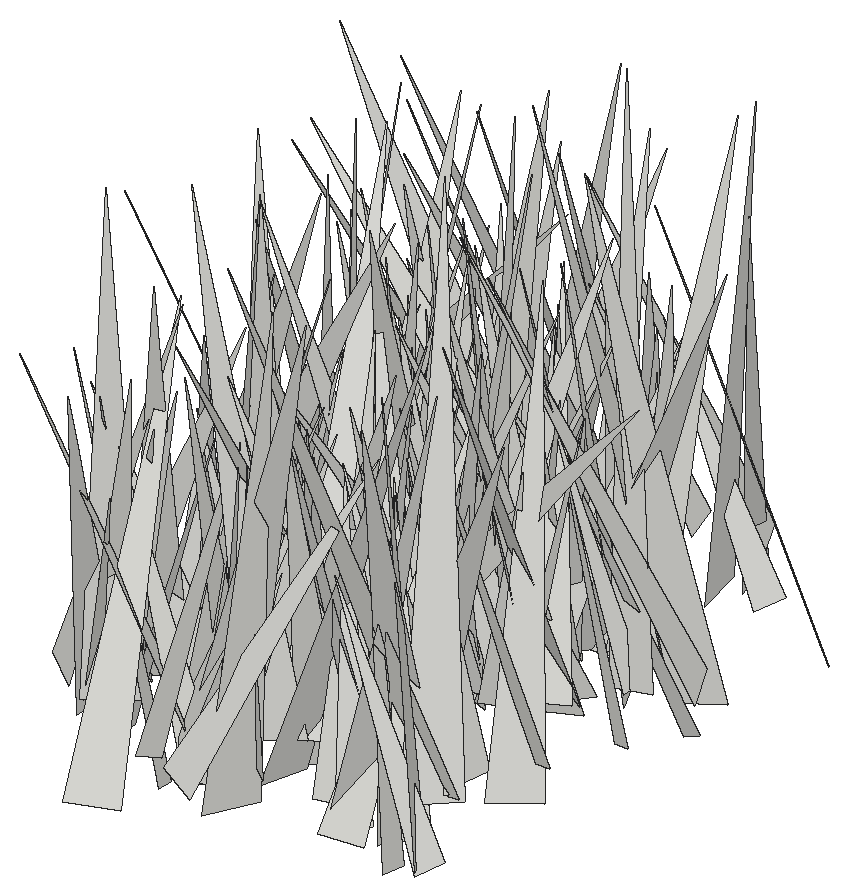
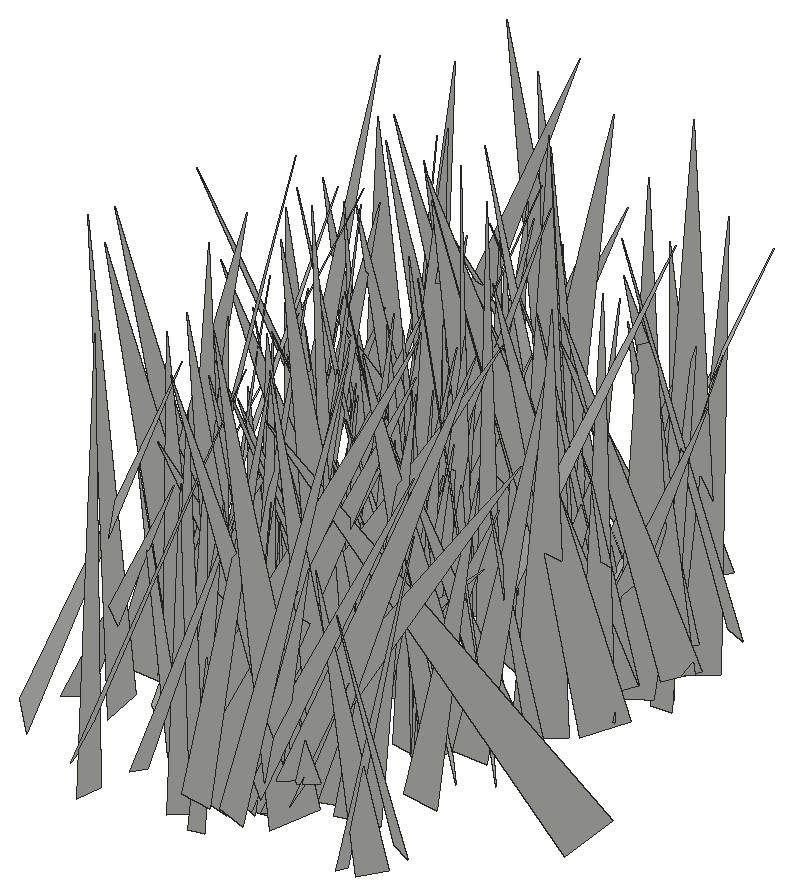
# SketchUp Ruby script. Lengths in inches.
U = 1.inch
M = Sketchup.active_model
def pt(a) = Geom::Point3d.new(a.map { |v| v * U })
def face(e, loops, mat)
  f = e.add_face(loops[0].map { |a| pt(a) })
  loops[1..].each { |l| e.add_face(l.map { |a| pt(a) }).erase! }
  f.material = f.back_material = mat if mat
  f
end
# faces: each face lists its corners as indices into pts; further lists are holes
def faces(e, pts, list, mat = nil) = list.each { |f| face(e, (f[0].is_a?(Array) ? f : [f]).map { |l| l.map { |i| pts[i] } }, mat) }
# xy, xz, yz: faces in a plane at the given z, y or x. An outline is a flat list of corners, or four numbers for a rectangle; further outlines are holes
def ring(l) = l.size == 4 ? [[l[0], l[1]], [l[2], l[1]], [l[2], l[3]], [l[0], l[3]]] : l.each_slice(2).to_a
def flat(e, list, mat, &to3) = list.each { |f| face(e, (f[0].is_a?(Array) ? f : [f]).map { |l| ring(l).map { |u, v| to3.(u, v) } }, mat) }
def xy(e, z, list, mat = nil) = flat(e, list, mat) { |x, y| [x, y, z] }
def xz(e, y, list, mat = nil) = flat(e, list, mat) { |x, z| [x, y, z] }
def yz(e, x, list, mat = nil) = flat(e, list, mat) { |y, z| [x, y, z] }
def lines(e, pts, list) = list.each { |a, b| e.add_line(pt(pts[a]), pt(pts[b])) }
# prism: a flat outline (further loops are holes) pulled along v
def prism(e, loops, v, mat = nil)
  f = face(e, loops, mat); d = Geom::Vector3d.new(v.map { |x| x * U })
  f.pushpull(f.normal.samedirection?(d) ? d.length : -d.length)
end
def box(e, o, s, mat = nil) = prism(e, [[o, [o[0] + s[0], o[1], o[2]], [o[0] + s[0], o[1] + s[1], o[2]], [o[0], o[1] + s[1], o[2]]]], [0, 0, s[2]], mat)
def at(x, y, z, deg = 0) = Geom::Transformation.translation(pt([x, y, z])) * Geom::Transformation.rotation(ORIGIN, Z_AXIS, deg.degrees)
def axes(o, x, y, z) = Geom::Transformation.new([*x, 0, *y, 0, *z, 0, *pt(o).to_a, 1])
def part(name) = M.definitions.add(name)
# library, detail: a bought-in or finely detailed component or shape, given as its bounding box
def library(name, o, s) = part(name).tap { |d| box(d.entities, o, s) }
def detail(e, o, s) = box(e.add_group.entities, o, s)
def put(e, d, t, mat = nil) = e.add_instance(d, t).tap { |i| i.material = mat if mat }
def group(e, t, mat = nil) = e.add_group.tap { |g| g.transformation = t; g.material = mat if mat }.entities
root = M.entities
c1 = part("fur_instance\#9")
p = [[0.8125,0,1.79],[0.67,-0.02,1.48],[0,-0.11,0],[0,0.11,0]]
faces(c1.entities,p,[[0,1,2,3]])
put(root,c1,axes([89.85,77.52,-28.22],[0.35019,4.61175,0.40741],[4.56098,-0.41379,0.76359],[-0.79477,-0.34263,4.56155]))
put(root,c1,axes([88.22,83.61,-27.1],[3.62066,0.28745,0.41277],[0.34104,-3.60783,-0.479],[-0.36973,-0.51296,3.60033]))
put(root,c1,axes([88.46,77.83,-28.22],[-1.94792,-5.41513,0.85515],[-5.11405,2.12183,1.78705],[1.97517,0.15336,5.47032]))
put(root,c1,axes([89.04,88.7,-28.22],[1.79566,3.71313,0.76849],[3.77743,-1.82574,-0.00496],[-0.33004,-0.69403,4.12452]))
put(root,c1,axes([90.1,81.2,-28.22],[-4.52139,5.22079,2.42729],[5.56937,4.74843,0.161],[1.45961,-1.94607,6.90462]))
put(root,c1,axes([91.15,77.77,-28.22],[-4.32688,2.05759,1.06704],[2.30248,4.07514,1.47851],[0.2661,-1.80382,4.55737]))
put(root,c1,axes([89.63,84.88,-27.1],[-0.57876,-6.04691,0.53315],[-6.05695,0.61084,0.35302],[0.40347,0.49606,6.06428]))
put(root,c1,axes([90.38,86.13,-28.22],[-0.10037,-5.00985,1.67679],[-5.24561,-0.10471,-0.62683],[-0.62754,1.67652,4.9715]))
put(root,c1,axes([87.71,81.27,-27.1],[5.60342,-3.67276,1.04707],[-3.81273,-5.48708,1.15708],[-0.22057,1.54484,6.59914]))
put(root,c1,axes([88.14,81.08,-27.1],[0.06322,-6.05576,0.15688],[-5.74231,-0.00994,1.93043],[1.92942,0.16885,5.74018]))
put(root,c1,axes([88.02,77.62,-27.1],[0.93957,-4.99379,0.05949],[-4.70596,-0.86502,1.71172],[1.67197,0.37157,4.78443]))
put(root,c1,axes([87.93,77.6,-27.1],[2.95683,-4.48742,1.40063],[-4.613,-2.45121,1.88504],[0.90496,2.16707,5.03253]))
put(root,c1,axes([88.21,74.84,-27.1],[3.54049,4.95211,1.34575],[5.12044,-3.30078,-1.32493],[0.33991,-1.85767,5.94164]))
put(root,c1,axes([89.72,90.47,-28.22],[-4.12038,-2.11418,1.50488],[-1.47976,4.23386,1.89649],[2.13184,-1.14743,4.225]))
put(root,c1,axes([88.83,75.66,-28.22],[6.03542,-2.39463,0.80521],[-2.12324,-5.9379,-1.74415],[-1.3691,-1.34759,6.25448]))
put(root,c1,axes([85.43,84.82,-28.22],[6.0984,-4.54505,0.22334],[-3.82324,-4.91501,4.37303],[2.46783,3.61705,6.22291]))
put(root,c1,axes([88.97,76.35,-27.1],[3.21186,-3.52218,0.8528],[-3.62385,-3.13,0.72104],[-0.02677,1.11644,4.71189]))
put(root,c1,axes([90.29,74.41,-27.1],[4.03772,-5.94106,3.0996],[-6.44975,-4.42725,-0.08397],[-1.8178,2.512,7.18278]))
put(root,c1,axes([89.54,74.5,-27.1],[3.73813,0.01426,0.67221],[0.17612,-3.68545,-0.90117],[-0.64889,-0.91811,3.62791]))
put(root,c1,axes([92.89,88.93,-28.22],[-7.69272,2.37823,1.5322],[2.71051,7.46743,2.01798],[0.8104,-2.40066,7.79498]))
put(root,c1,axes([89.15,77.73,-28.22],[4.02071,-6.30995,0.86141],[-6.36147,-4.02715,0.19326],[-0.29869,0.83076,7.47959]))
put(root,c1,axes([92.9,73.3,-28.22],[-5.46466,-2.11839,0.66349],[-2.21236,5.05235,-2.09036],[-0.18243,2.18553,5.47545]))
put(root,c1,axes([88.9,90.13,-28.22],[2.31724,-3.70248,0.25487],[-3.62607,-2.19471,1.08527],[0.79054,0.78602,4.23086]))
put(root,c1,axes([94.19,88.4,-28.22],[-2.35699,-6.63901,0.53799],[-6.01099,1.87426,-3.2057],[-2.86948,1.52709,6.27339]))
put(root,c1,axes([89.55,75.04,-27.1],[3.84963,-3.94903,0.87916],[-4.01863,-3.87266,0.20133],[-0.4673,0.77142,5.51126]))
put(root,c1,axes([89.84,83.51,-28.22],[5.88152,4.86813,2.28116],[5.13014,-6.09312,-0.22398],[-1.60749,-1.63397,7.63157]))
put(root,c1,axes([90.27,75.01,-28.22],[4.03699,1.00135,1.00845],[0.75439,-4.0837,1.03503],[-1.2044,0.79854,4.02849]))
put(root,c1,axes([93.26,80.22,-27.1],[-4.92734,-5.46841,0.2776],[-5.45988,4.87887,-0.80338],[-0.41255,0.74316,7.31688]))
put(root,c1,axes([93.45,89.71,-27.1],[-3.66042,-4.84933,0.70173],[-4.78346,3.34689,-1.82316],[-1.06154,1.63996,5.79575]))
put(root,c1,axes([89.6,83.15,-27.1],[4.44559,-0.41699,0.42413],[-0.48383,-4.39553,0.74982],[-0.34594,0.78895,4.4017]))
put(root,c1,axes([93.32,74.62,-28.22],[-5.39414,-3.77764,0.22745],[-3.78403,5.38986,-0.22257],[0.05845,0.31282,6.58162]))
put(root,c1,axes([91.07,88.09,-28.22],[1.80262,-6.00522,1.15434],[-6.08405,-1.88243,-0.2921],[-0.61598,1.01901,6.26312]))
put(root,c1,axes([91.19,76.49,-28.22],[3.26782,5.25044,1.3347],[5.28581,-3.43164,0.55786],[-1.18691,-0.82697,6.1591]))
put(root,c1,axes([92.125,71.23,-28.22],[-4.33285,5.33033,0.39838],[5.19442,4.31986,-1.30443],[1.26061,0.52067,6.74422]))
put(root,c1,axes([91.43,83.35,-28.22],[-4.86903,5.31705,1.90275],[5.12727,5.21523,-1.45307],[2.36698,-0.35954,7.06166]))
put(root,c1,axes([93.01,77.57,-28.22],[-1.35537,3.98703,1.26023],[4.07237,0.95801,1.34893],[-0.94888,-1.58348,3.98921]))
put(root,c1,axes([91.51,77.72,-27.1],[4.6906,-0.13116,1.94102],[0.35682,-4.92253,-1.19491],[-1.91244,-1.24013,4.53774]))
put(root,c1,axes([92.78,88.86,-28.22],[-3.67924,-0.76157,0.35539],[-0.68587,3.64327,0.70657],[0.48566,-0.62424,3.6902]))
put(root,c1,axes([93.61,81.77,-27.1],[-2.38468,3.13652,0.12042],[3.02513,2.25628,1.13874],[-0.83714,-0.7813,3.77197]))
put(root,c1,axes([93.64,73.99,-28.22],[-2.38269,3.95567,1.05235],[4.03891,2.07425,1.34786],[-0.66484,-1.57548,4.41677]))
put(root,c1,axes([90.74,84.18,-28.22],[-4.56158,-4.36485,4.54967],[-5.17144,5.80258,0.38189],[3.60662,2.79958,6.30192]))
put(root,c1,axes([88.87,79.65,-27.1],[4.47531,-6.51665,1.20055],[-6.35255,-3.80729,3.0143],[1.88498,2.64087,7.30815]))
put(root,c1,axes([92.51,84.03,-28.22],[-3.25997,-4.21096,1.97124],[-4.4396,3.53441,0.20814],[1.38129,1.42168,5.3213]))
put(root,c1,axes([92.71,91.65,-27.1],[-2.90954,-6.16313,0.64564],[-6.10361,2.97343,0.8781],[1.07095,0.20243,6.75859]))
put(root,c1,axes([93.57,84.49,-28.22],[-6.39617,-0.72322,1.67284],[-0.5993,6.59982,0.56183],[1.72113,-0.38959,6.41236]))
put(root,c1,axes([93.48,89.43,-28.22],[1.42744,-3.53628,2.17287],[-3.81125,-2.02664,-0.79456],[-1.64348,1.62839,3.72982]))
put(root,c1,axes([92.29,80.73,-28.22],[7.19679,1.10507,2.93039],[1.40985,-7.70082,-0.55845],[-2.79655,-1.03845,7.25969]))
put(root,c1,axes([92.34,85.6,-28.22],[4.23333,1.58778,2.03705],[2.11026,-4.38143,-0.97034],[-1.48911,-1.69519,4.41595]))
put(root,c1,axes([92.1,78.51,-27.1],[3.60415,-6.43604,2.10161],[-6.7075,-3.71823,0.11619],[-0.92131,1.89247,7.37557]))
put(root,c1,axes([89.6875,79.16,-28.22],[8.03575,1.73258,0.69022],[1.85682,-7.7181,-2.24381],[-0.17451,-2.34107,7.90825]))
put(root,c1,axes([96.3,86.22,-27.1],[-7.10232,2.48969,0.17848],[2.39972,6.66255,2.55443],[-0.68683,-2.46683,7.07929]))
put(root,c1,axes([92.89,72.65,-27.1],[-4.41851,1.16155,1.66424],[0.34777,4.36157,-2.12081],[1.99949,1.8082,4.04655]))
put(root,c1,axes([92.1,83.53,-28.22],[5.9168,-1.45412,1.7202],[-1.44139,-6.15974,-0.24915],[-1.73089,0.15879,6.08776]))
put(root,c1,axes([92.58,84.09,-28.22],[-1.22041,-5.00142,1.71972],[-5.19067,1.47111,0.5948],[1.01418,1.51086,5.11369]))
put(root,c1,axes([95.125,89.82,-28.22],[0.03934,-7.1777,0.79174],[-6.87762,-0.27857,-2.18369],[-2.20103,0.74216,6.83757]))
put(root,c1,axes([92.08,87.73,-28.22],[0.14436,6.2225,2.72909],[6.68972,0.34776,-1.14678],[1.18962,-2.71069,6.11762]))
put(root,c1,axes([93.19,78.625,-28.22],[-1.7362,-3.80786,1.79903],[-4.13168,1.91701,0.07019],[0.81577,1.60498,4.18441]))
put(root,c1,axes([96.39,82.44,-28.22],[-3.03964,-3.22245,0.08473],[-2.53096,2.3136,-2.80576],[-1.9964,1.97328,3.42802]))
put(root,c1,axes([92.57,80.72,-27.1],[3.35621,4.76804,0.53975],[4.75729,-3.3924,0.38655],[-0.62744,-0.21695,5.81798]))
put(root,c1,axes([93.99,85.64,-28.22],[-1.52023,5.3398,1.43684],[5.52962,1.4775,0.35965],[0.03531,-1.48075,5.54032]))
put(root,c1,axes([93.42,80.28,-27.1],[4.5767,5.68819,3.18986],[6.17982,-5.02762,0.09872],[-2.08339,-2.41752,7.30013]))
put(root,c1,axes([92.99,77.04,-27.1],[2.64907,4.14771,0.84835],[4.17625,-2.72433,0.27885],[-0.69438,-0.56151,4.91358]))
put(root,c1,axes([96.71,88.74,-28.22],[-3.02685,-7.70536,1.30124],[-7.48247,2.45538,-2.86554],[-2.25353,2.19686,7.76679]))
put(root,c1,axes([93.05,81.78,-27.1],[3.48904,-1.79502,0.75996],[-1.60226,-3.52839,-0.97792],[-1.11014,-0.54905,3.7999]))
put(root,c1,axes([94.92,75.38,-27.1],[1.79805,-6.87497,3.712],[-7.43664,-2.674,-1.35027],[-2.39594,3.14033,6.97674]))
put(root,c1,axes([94.07,74.16,-28.22],[-7.10447,-2.39928,3.44832],[-3.25719,7.42464,-1.54476],[2.65295,2.69055,7.33783]))
put(root,c1,axes([95.2,80.11,-27.1],[-4.58169,-0.00231,0.33908],[-0.10273,4.38765,-1.35823],[0.32316,1.36211,4.37574]))
put(root,c1,axes([93.87,89.46,-28.22],[-1.43466,-3.23484,0.82707],[-3.31328,1.49057,0.08262],[0.41278,0.72144,3.53774]))
put(root,c1,axes([93.36,81.81,-27.1],[0.28978,-3.77503,0.68612],[-3.83038,-0.24462,0.27184],[0.22308,0.70349,3.77636]))
put(root,c1,axes([92.47,89.13,-28.22],[7.15421,-1.9799,2.12173],[-2.22149,-7.36827,0.61487],[-1.86728,1.18029,7.39761]))
put(root,c1,axes([95.91,78,-28.22],[-0.66678,7.09806,0.59701],[6.83624,0.46921,2.05647],[-2.00116,-0.76214,6.82627]))
put(root,c1,axes([94.06,91.54,-27.1],[-1.823,-5.96341,0.88128],[-5.94354,1.93183,0.77754],[1.00658,0.60664,6.18716]))
put(root,c1,axes([96.38,80.29,-28.22],[-7.8071,-1.03462,1.04066],[-0.93299,7.84786,0.80297],[1.13267,-0.66693,7.83431]))
put(root,c1,axes([93.01,86.04,-27.1],[-2.73382,6.12597,3.74599],[6.6709,3.64992,-1.10045],[2.6569,-2.86083,6.61742]))
put(root,c1,axes([92.61,85.71,-27.1],[1.69765,-3.69471,0.41656],[-3.54176,-1.46758,1.41724],[1.13153,0.9496,3.81108]))
put(root,c1,axes([96.04,78.1,-27.1],[-1.10699,-6.38687,0.31821],[-6.26084,1.01671,-1.37367],[-1.30201,0.54128,6.33487]))
put(root,c1,axes([92.375,88.9375,-27.1],[1.25839,-5.65908,2.69216],[-6.0262,-0.33916,2.10388],[1.71982,2.95233,5.40207]))
put(root,c1,axes([95.6,75.94,-27.1],[-4.43994,6.98412,0.3729],[6.94517,4.45476,-0.74146],[0.82561,0.08476,8.24265]))
put(root,c1,axes([96.21,78.95,-27.1],[-2.14589,-4.13922,0.79032],[-4.13009,1.88974,-1.31675],[-0.83673,1.28775,4.4726]))
put(root,c1,axes([94.56,80.97,-27.1],[3.67967,2.76321,1.03507],[2.46473,-3.78797,1.35021],[-1.62229,0.51247,4.39911]))
put(root,c1,axes([93.76,82.29,-27.1],[0.23103,-4.99246,1.62863],[-5.17408,0.0623,0.92493],[0.89778,1.64376,4.91147]))
put(root,c1,axes([93.25,83.4375,-27.1],[6.31463,-5.10403,0.36931],[-4.97216,-6.25818,-1.47472],[-1.21044,-0.91981,7.98441]))
put(root,c1,axes([92.95,73.8,-27.1],[3.70587,4.25797,0.60198],[4.28884,-3.60158,-0.92773],[0.31394,-1.06043,5.56805]))
put(root,c1,axes([94.41,73.7,-27.1],[1.13394,4.06883,0.24777],[4.07369,-1.14042,0.08414],[-0.14769,-0.216,4.22305]))
put(root,c1,axes([93.99,87.58,-28.22],[3.64013,-0.49009,0.65042],[-0.33955,-3.62113,-0.82821],[-0.74023,-0.74902,3.57838]))
put(root,c1,axes([93.8125,74.01,-28.22],[4.14579,-2.60609,2.17076],[-3.31381,-3.84297,1.71517],[-0.72292,2.67047,4.58667]))
put(root,c1,axes([96.46,77.41,-28.22],[-5.48359,2.23586,1.70204],[2.68404,5.27249,1.72124],[0.83185,-2.27324,5.66623]))
put(root,c1,axes([93.81,78.3,-27.1],[5.31663,-1.02418,0.76649],[-0.77202,-5.18142,-1.56841],[-1.02002,-1.41668,5.18224]))
put(root,c1,axes([94.58,74.5,-27.1],[3.50873,2.55931,1.93983],[3.03472,-3.58228,-0.76287],[-1.05048,-1.80039,4.27543]))
put(root,c1,axes([95.61,81.625,-28.22],[3.52477,-3.78027,2.43443],[-3.94318,-4.08529,-0.63451],[-2.1606,1.28874,5.1295]))
put(root,c1,axes([97.88,79.3,-28.22],[-1.67581,5.69721,1.32161],[5.39716,0.9769,2.63242],[-2.25291,-1.89755,5.32325]))
put(root,c1,axes([96.53,86.07,-27.1],[-0.29394,-4.28793,0.2812],[-4.0742,0.18848,-1.38464],[-1.36614,0.36048,4.06885]))
put(root,c1,axes([96.42,81.74,-28.22],[-3.5063,-5.04513,2.56803],[-5.65565,3.25438,-1.32851],[0.24851,2.88062,5.99854]))
put(root,c1,axes([95.85,83.48,-27.1],[-3.35833,-3.2337,1.73378],[-3.57177,3.41915,-0.54142],[0.83981,1.61055,4.63056]))
put(root,c1,axes([94.2,91.33,-28.22],[3.64505,-0.39812,0.27738],[-0.20845,-3.18305,-1.82936],[-0.43816,-1.79764,3.17779]))
put(root,c1,axes([95.62,73.77,-27.1],[-2.49049,-3.07283,1.62396],[-3.33154,2.67981,-0.03854],[0.99012,1.28779,3.95516]))
put(root,c1,axes([96.83,80.66,-28.22],[-3.33504,1.53851,0.16438],[1.54705,3.32218,0.29368],[0.02564,-0.33558,3.66104]))
put(root,c1,axes([96.35,87.49,-27.1],[-3.41179,-1.77285,0.16017],[-1.67154,3.30984,1.02951],[0.61205,-0.84317,3.70451]))
put(root,c1,axes([95.3,87.68,-28.22],[-2.68709,-2.60275,1.28992],[-2.48203,2.97011,0.82256],[1.50922,0.25052,3.6494]))
put(root,c1,axes([94.3,78.03,-27.1],[-0.53016,-5.209,0.61736],[-4.97847,0.69512,1.58982],[1.65216,0.4231,4.98871]))
put(root,c1,axes([95.52,84.36,-27.1],[2.55514,-3.36467,0.69917],[-3.31318,-2.64324,-0.61213],[-0.91251,0.1757,4.18031]))
put(root,c1,axes([96.38,91.1875,-27.1],[-4.22859,-0.79072,0.99748],[-0.41595,4.12901,1.5098],[1.20299,-1.35177,4.02824]))
put(root,c1,axes([95.66,89.77,-27.1],[0.8315,-3.67241,0.7269],[-3.73531,-0.86356,-0.09004],[-0.24991,0.6885,3.76429]))
put(root,c1,axes([95.02,73.39,-28.22],[6.93717,-2.75986,2.51351],[-2.97128,-7.29338,0.19237],[-2.25967,1.11744,7.46352]))
put(root,c1,axes([95.38,76.72,-28.22],[3.36896,-5.0045,1.18358],[-5.04079,-3.49374,-0.42432],[-1.01802,0.73793,6.01788]))
put(root,c1,axes([96.93,83.9375,-27.1],[-5.40914,1.11965,1.3835],[1.23539,5.5484,0.3398],[1.28121,-0.62292,5.51334]))
put(root,c1,axes([93.54,74.89,-27.1],[5.39011,-5.98506,0.75501],[-6.02641,-5.29691,1.03406],[0.27067,1.25142,7.9878]))
put(root,c1,axes([94.32,80.53,-28.22],[3.5807,5.01538,0.32607],[5.01642,-3.54168,-0.61141],[0.30977,-0.61982,6.13202]))
put(root,c1,axes([93.57,77.95,-28.22],[3.71453,-6.09838,0.78607],[-6.05056,-3.46164,1.73599],[1.09493,1.55972,6.92635]))
put(root,c1,axes([95.15,83.68,-28.22],[4.01305,-1.4697,0.35123],[-1.33059,-3.90931,-1.15533],[-0.71618,-0.97223,4.11458]))
put(root,c1,axes([96.84,81.49,-27.1],[-5.64756,-4.03637,0.24701],[-3.60758,5.22048,2.82493],[1.82721,-2.16853,6.3409]))
put(root,c1,axes([95.04,90.76,-28.22],[3.21105,-3.45107,0.18225],[-3.45172,-3.21492,-0.06213],[-0.16965,0.09106,4.71348]))
put(root,c1,axes([96.62,82.15,-27.1],[3.17531,6.56755,2.54139],[6.79761,-3.58673,0.77578],[-1.83954,-1.91744,7.25351]))
put(root,c1,axes([95.5,89.71,-27.1],[-0.07367,-4.26522,0.50041],[-4.16979,0.19077,1.01214],[1.02732,0.46845,4.14405]))
put(root,c1,axes([95.33,90.36,-27.1],[0.2797,-5.08952,0.70223],[-5.01624,-0.11848,1.13926],[1.11073,0.74654,4.96825]))
put(root,c1,axes([94.34,71.99,-27.1],[1.81357,5.35205,0.20733],[5.12174,-1.66889,-1.72019],[1.56691,-0.73948,5.38279]))
put(root,c1,axes([97.3125,80.56,-27.1],[-0.77658,-4.10323,1.17838],[-4.23531,0.59015,-0.73621],[-0.53592,1.28194,4.11067]))
put(root,c1,axes([97.63,76.18,-28.22],[-2.42816,-5.42807,1.43938],[-5.61543,2.33238,-0.67728],[-0.05217,1.5899,5.90772]))
put(root,c1,axes([97.05,75.31,-28.22],[-1.64071,6.20292,1.41522],[6.35653,1.66047,0.09149],[0.27128,-1.39198,6.41559]))
put(root,c1,axes([95.48,85.72,-27.1],[5.08569,0.11573,0.95874],[0.07501,-5.17107,0.22632],[-0.96278,0.20845,5.08197]))
put(root,c1,axes([98.34,83.42,-28.22],[1.14957,-5.99203,1.40359],[-5.68779,-1.57972,-2.08556],[-2.35023,0.89221,5.73379]))
put(root,c1,axes([98.45,76.41,-28.22],[-5.17368,4.83178,0.63052],[4.85594,5.1888,0.08232],[0.40437,-0.49072,7.07858]))
put(root,c1,axes([98.26,91.62,-27.1],[-5.70608,-2.81682,0.48614],[-2.67601,5.6456,1.30244],[1.0049,-0.96065,6.22877]))
put(root,c1,axes([96.73,86.46,-27.1],[-3.34858,-4.98605,1.16696],[-4.83329,3.53804,1.24784],[1.69169,0.23891,5.87509]))
put(root,c1,axes([97.04,78.9,-27.1],[-3.71631,2.59474,2.95715],[3.6126,3.86147,1.15179],[1.55775,-2.76492,4.38373]))
put(root,c1,axes([95.0625,82.93,-28.22],[2.79379,4.96818,0.70977],[4.95175,-2.59669,-1.31495],[0.8165,-1.25148,5.54607]))
put(root,c1,axes([96.2,77.72,-28.22],[5.43956,-0.0104,1.6458],[0.01524,-5.68242,-0.08629],[-1.64576,-0.087,5.43889]))
put(root,c1,axes([97.13,85.77,-28.22],[-1.01475,7.09695,1.79918],[7.31311,1.06925,-0.09303],[0.3496,-1.76734,7.16853]))
put(root,c1,axes([95.45,83.1875,-27.1],[4.11337,-1.35782,0.42666],[-1.42017,-4.00175,0.95638],[-0.09392,1.04301,4.22479]))
put(root,c1,axes([96.54,85.43,-28.22],[-1.17903,-5.46423,1.73554],[-5.62366,1.44698,0.7353],[1.11548,1.51937,5.54141]))
put(root,c1,axes([98.17,74.54,-28.22],[-4.11869,2.39634,0.55767],[2.352,4.15398,-0.47915],[0.72219,0.13795,4.74094]))
put(root,c1,axes([95.05,75.52,-28.22],[7.44021,-1.05618,0.97458],[-1.13327,-7.472,0.55406],[-0.88376,0.68976,7.49435]))
put(root,c1,axes([95.67,81.49,-28.22],[-0.17372,7.00266,1.70424],[6.95108,0.61311,-1.81067],[1.90374,-1.5996,6.76675]))
put(root,c1,axes([96.63,78.625,-28.22],[4.55576,-0.64185,1.19418],[-0.37344,-4.61891,-1.05794],[-1.3033,-0.92017,4.47746]))
put(root,c1,axes([97.33,79.07,-27.1],[4.31579,6.0344,1.65644],[5.97789,-4.5707,1.07586],[-1.85004,-0.69181,7.34048]))
put(root,c1,axes([97.5,76.57,-28.22],[0.08321,7.29137,1.2347],[7.39423,-0.10178,0.10277],[-0.11831,-1.23331,7.29112]))
put(root,c1,axes([96.82,79.28,-27.1],[3.38987,-1.12165,1.00676],[-1.27426,-3.45624,0.43994],[-0.80492,0.7478,3.54341]))
put(root,c1,axes([98.49,81.03,-27.1],[5.38161,2.47127,3.67462],[2.66712,-6.4254,0.41515],[-3.53503,-1.08568,5.90733]))
put(root,c1,axes([97.625,77.54,-27.1],[3.16597,-2.82128,1.36449],[-2.73379,-3.43456,-0.75836],[-1.53229,0.2984,4.17228]))
put(root,c1,axes([99.97,75.83,-27.1],[-2.55131,-7.67351,1.38924],[-7.65133,2.18082,-2.00574],[-1.50657,1.91917,7.83383]))
put(root,c1,axes([96.98,87.5,-27.1],[3.24454,-4.71501,1.03025],[-4.7617,-3.32972,-0.24278],[-0.78672,0.70811,5.71834]))
put(root,c1,axes([96.15,89.81,-27.1],[4.14097,0.37336,0.37849],[0.46882,-3.96604,-1.21698],[-0.25072,-1.24957,3.97567]))
put(root,c1,axes([96.62,83.65,-28.22],[4.77554,-0.30271,1.03368],[-0.19329,-4.86277,-0.53104],[-1.0596,-0.47722,4.75556]))
put(root,c1,axes([98.83,80.36,-28.22],[-5.33411,1.7362,0.45715],[1.45522,5.02033,-2.08679],[1.05153,1.85957,5.20696]))
put(root,c1,axes([96.3125,80.91,-27.1],[-1.36067,-5.7583,1.83351],[-5.61411,1.9,1.80082],[2.23642,1.26617,5.63617]))
put(root,c1,axes([98.22,79.11,-28.22],[-2.7828,-3.97435,1.2381],[-4.07565,2.90431,0.16237],[0.84701,0.91751,4.84903]))
put(root,c1,axes([98.43,82.6,-28.22],[1.44091,-6.85532,1.40735],[-6.89305,-1.6385,-0.92385],[-1.20912,1.1714,6.94393]))
put(root,c1,axes([96.79,84.88,-28.22],[3.8804,-2.67072,0.47699],[-2.66948,-3.90717,-0.15997],[-0.48385,0.13783,4.70793]))
put(root,c1,axes([98.09,78.16,-27.1],[2.45481,-4.16097,0.8917],[-4.06011,-2.59844,-0.9479],[-1.27449,0.26329,4.73722]))
put(root,c1,axes([98.3,73.84,-28.22],[-4.56686,4.07542,0.09193],[3.68922,4.19072,-2.51023],[1.73411,1.8173,5.58247]))
put(root,c1,axes([97.34,83.68,-27.1],[-2.89965,3.32427,1.06428],[2.78447,3.03733,-1.90073],[2.1048,0.5615,3.98069]))
put(root,c1,axes([99.96,75.53,-27.1],[-1.66543,4.2087,0.7623],[4.0491,1.28782,1.73616],[-1.37806,-1.30242,4.18002]))
put(root,c1,axes([99.22,81.3,-27.1],[-1.93628,5.55,0.46539],[5.55779,1.89356,0.54185],[-0.36056,-0.61659,5.85304]))
put(root,c1,axes([98,83.71,-27.1],[-0.65259,-3.58567,0.77528],[-3.62638,0.74954,0.41412],[0.55447,0.682,3.62097]))
put(root,c1,axes([99.67,85.85,-27.1],[-7.3935,-3.44968,1.78048],[-3.41196,7.60131,0.55924],[1.85173,0.23234,8.13949]))
put(root,c1,axes([98.94,78.67,-28.22],[-3.6032,0.74818,1.09352],[0.87855,3.72087,0.34907],[0.99182,-0.57787,3.66346]))
put(root,c1,axes([100.46,83.15,-27.1],[1.13757,8.04859,1.54719],[7.76789,-1.55698,2.3882],[-2.61411,-1.12413,7.76984]))
put(root,c1,axes([100.15,75.3,-27.1],[-7.18499,4.19207,1.05141],[4.04317,7.24035,-1.23823],[1.52698,0.55406,8.22584]))
put(root,c1,axes([99.71,75,-28.22],[-3.61656,3.24074,0.55892],[3.26072,3.64166,-0.01623],[0.42715,-0.36083,4.85609]))
put(root,c1,axes([99.27,84.58,-28.22],[-5.57513,-2.9786,1.92177],[-3.03694,5.86084,0.2736],[1.82819,0.65252,6.315]))
put(root,c1,axes([99.23,74.52,-28.22],[-3.69275,-0.52533,1.17947],[-0.76187,3.77166,-0.70545],[1.04243,0.89562,3.66261]))
put(root,c1,axes([98.05,87.1,-27.1],[4.42383,-2.92058,1.2942],[-2.99041,-4.56361,-0.07677],[-1.12348,0.64702,5.30039]))
put(root,c1,axes([100.41,88.97,-27.1],[-3.73947,1.85603,0.44676],[1.90802,3.6015,1.00834],[-0.06253,-1.10111,4.05114]))
put(root,c1,axes([99.38,86.73,-28.22],[-5.6893,-5.57398,0.54513],[-5.22917,5.56506,2.3282],[2.00554,-1.30211,7.61688]))
put(root,c1,axes([100.33,73.47,-28.22],[-5.41908,-0.82486,1.13145],[-1.12996,5.24719,-1.58656],[0.82691,1.76453,5.24687]))
put(root,c1,axes([96.31,79.47,-28.22],[3.61715,-5.66391,0.01487],[-5.50634,-3.51236,1.58351],[1.3268,0.86448,6.53117]))
put(root,c1,axes([97.92,91.49,-28.22],[6.38697,0.74513,2.00431],[1.2691,-6.40204,-1.66407],[-1.72101,-1.95564,6.21124]))
put(root,c1,axes([97.92,74.54,-28.22],[6.43486,-0.85229,1.84553],[-1.08084,-6.62327,0.70985],[-1.72168,0.97247,6.45212]))
put(root,c1,axes([98.2,80.37,-27.1],[2.26375,-3.28304,0.92587],[-3.40814,-2.22313,0.4499],[-0.14199,1.01955,3.96238]))
put(root,c1,axes([94.0625,81.42,-27.1],[5.26826,5.58359,0.80335],[4.69893,-3.73546,-4.8521],[3.1212,-3.80083,5.9488]))
put(root,c1,axes([100.41,83.36,-27.1],[-3.8674,0.14725,0.40736],[0.1724,3.88071,0.23399],[0.39736,-0.25058,3.86312]))
put(root,c1,axes([98.27,76.68,-27.1],[2.21636,-6.61774,0.25451],[-6.61771,-2.20273,0.35418],[0.25535,0.35358,6.97003]))
put(root,c1,axes([101.76,84.43,-27.1],[-6.74137,-3.47517,0.05647],[-3.44773,6.70195,0.85032],[0.43951,-0.73012,7.53656]))
put(root,c1,axes([101.05,74.1,-28.22],[-3.99444,1.28958,0.25526],[1.31279,3.95594,0.55757],[0.06915,-0.60932,4.16025]))
put(root,c1,axes([99.3,84.8125,-27.1],[-5.55671,4.70477,2.20019],[4.40361,5.97611,-1.65743],[2.7539,-0.06297,7.08977]))
put(root,c1,axes([100.99,85.28,-28.22],[1.07794,-7.21694,3.00432],[-7.53412,-1.768,-1.54384],[-2.08502,2.65746,7.13181]))
put(root,c1,axes([101.94,83.84,-28.22],[-2.15609,-3.98258,0.83043],[-3.73233,1.56246,-2.1972],[-1.61872,1.70208,3.96005]))
put(root,c1,axes([99.72,80.4,-27.1],[-3.13954,-2.86345,1.03549],[-2.74612,3.30524,0.81394],[1.31545,0.06589,4.17056]))
put(root,c1,axes([101.12,78.62,-27.1],[-2.05485,-3.90462,0.97999],[-3.96047,1.76344,-1.27819],[-0.72186,1.43981,4.22312]))
put(root,c1,axes([98.98,88.68,-27.1],[7.15031,1.42356,2.57616],[1.59453,-7.56218,-0.24693],[-2.47399,-0.75958,7.28646]))
put(root,c1,axes([100.84,82.28,-28.22],[0.98464,3.25356,1.70885],[3.23357,-1.6077,1.19779],[-1.74639,-1.14237,3.18127]))
put(root,c1,axes([102.05,89.22,-28.22],[-4.77204,-4.71706,0.72174],[-4.75307,4.60775,-1.31181],[-0.42413,1.43592,6.58044]))
put(root,c1,axes([98.78,80.63,-27.1],[2.69077,3.3772,1.27263],[3.60609,-2.57991,-0.77814],[-0.14558,-1.48455,4.24737]))
put(root,c1,axes([100.55,74.3,-28.22],[-5.61783,-2.93903,2.21928],[-3.25584,5.85535,-0.48739],[1.72124,1.48327,6.32142]))
put(root,c1,axes([100.58,78.2,-28.22],[-4.66477,5.25581,1.41142],[5.28211,4.8201,-0.49149],[1.30953,-0.72026,7.01013]))
put(root,c1,axes([98.83,82.34,-27.1],[-2.64275,-7.72517,0.10148],[-7.35563,2.5487,2.46402],[2.36287,-0.70608,7.78402]))
put(root,c1,axes([97.01,85.73,-28.22],[6.73019,-3.63445,0.24466],[-3.63894,-6.68481,0.79754],[0.16506,0.81773,7.60715]))
